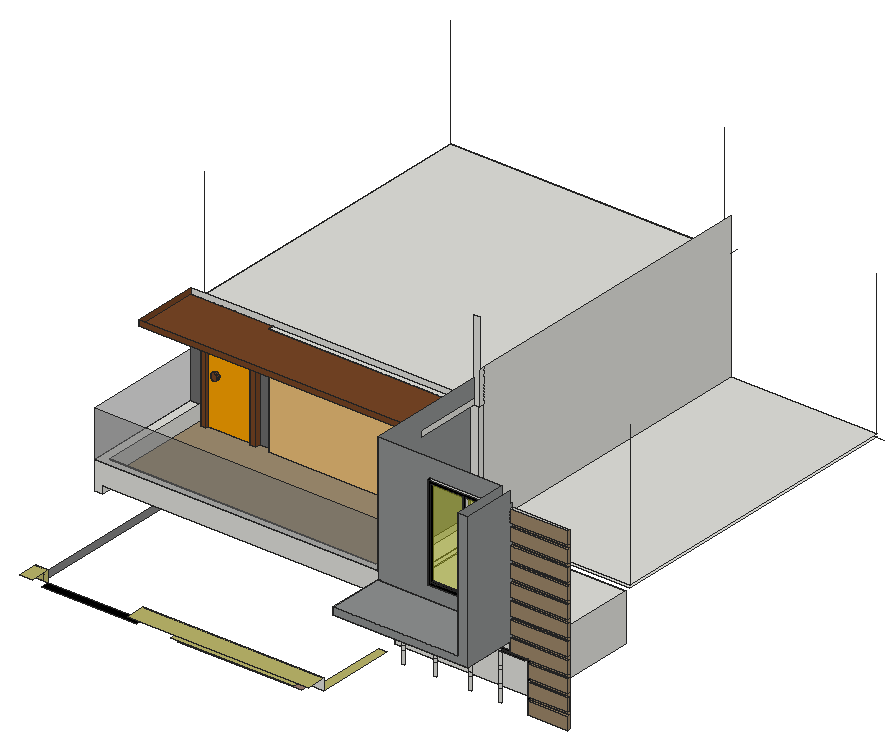
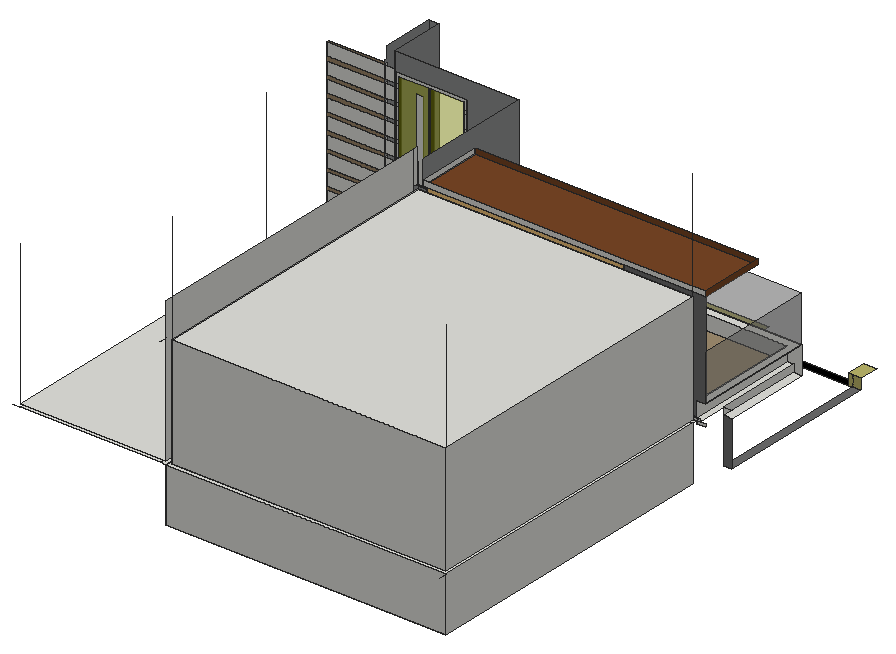
# SketchUp Ruby script. Lengths in inches.
U = 1.inch
M = Sketchup.active_model
def pt(a) = Geom::Point3d.new(a.map { |v| v * U })
def face(e, loops, mat)
  f = e.add_face(loops[0].map { |a| pt(a) })
  loops[1..].each { |l| e.add_face(l.map { |a| pt(a) }).erase! }
  f.material = f.back_material = mat if mat
  f
end
# faces: each face lists its corners as indices into pts; further lists are holes
def faces(e, pts, list, mat = nil) = list.each { |f| face(e, (f[0].is_a?(Array) ? f : [f]).map { |l| l.map { |i| pts[i] } }, mat) }
# xy, xz, yz: faces in a plane at the given z, y or x. An outline is a flat list of corners, or four numbers for a rectangle; further outlines are holes
def ring(l) = l.size == 4 ? [[l[0], l[1]], [l[2], l[1]], [l[2], l[3]], [l[0], l[3]]] : l.each_slice(2).to_a
def flat(e, list, mat, &to3) = list.each { |f| face(e, (f[0].is_a?(Array) ? f : [f]).map { |l| ring(l).map { |u, v| to3.(u, v) } }, mat) }
def xy(e, z, list, mat = nil) = flat(e, list, mat) { |x, y| [x, y, z] }
def xz(e, y, list, mat = nil) = flat(e, list, mat) { |x, z| [x, y, z] }
def yz(e, x, list, mat = nil) = flat(e, list, mat) { |y, z| [x, y, z] }
def lines(e, pts, list) = list.each { |a, b| e.add_line(pt(pts[a]), pt(pts[b])) }
# prism: a flat outline (further loops are holes) pulled along v
def prism(e, loops, v, mat = nil)
  f = face(e, loops, mat); d = Geom::Vector3d.new(v.map { |x| x * U })
  f.pushpull(f.normal.samedirection?(d) ? d.length : -d.length)
end
def box(e, o, s, mat = nil) = prism(e, [[o, [o[0] + s[0], o[1], o[2]], [o[0] + s[0], o[1] + s[1], o[2]], [o[0], o[1] + s[1], o[2]]]], [0, 0, s[2]], mat)
def at(x, y, z, deg = 0) = Geom::Transformation.translation(pt([x, y, z])) * Geom::Transformation.rotation(ORIGIN, Z_AXIS, deg.degrees)
def axes(o, x, y, z) = Geom::Transformation.new([*x, 0, *y, 0, *z, 0, *pt(o).to_a, 1])
def part(name) = M.definitions.add(name)
# library, detail: a bought-in or finely detailed component or shape, given as its bounding box
def library(name, o, s) = part(name).tap { |d| box(d.entities, o, s) }
def detail(e, o, s) = box(e.add_group.entities, o, s)
def put(e, d, t, mat = nil) = e.add_instance(d, t).tap { |i| i.material = mat if mat }
def group(e, t, mat = nil) = e.add_group.tap { |g| g.transformation = t; g.material = mat if mat }.entities
root = M.entities
M.materials.add("Niraj_Hair_Dark").color = [109, 109, 109]
M.materials.add("Niraj_Skin").color = [158, 128, 115]
M.materials.add("[0035_Tan]").color = [158, 135, 105]
M.materials.add("[0038_Orange]").color = [255, 165, 0]
M.materials.add("[0057_DarkKhaki]").color = [189, 183, 107]
M.materials.add("[0137_Black]").color = [0, 0, 0]
M.materials.add("[Blacktop Old 02]").color = [143, 145, 145]
M.materials.add("[Tile Border Travertine]").color = [160, 142, 112]
M.materials.add("[Translucent Glass Gray]").color = [198, 206, 26]
M.materials["[Translucent Glass Gray]"].alpha = 0.5
M.materials.add("[Translucent Glass Gray]1").color = [128, 128, 128]
M.materials["[Translucent Glass Gray]1"].alpha = 0.5
M.materials.add("[Wood OSB]").color = [240, 195, 122]
M.materials.add("[Wood Veneer 01]").color = [120, 70, 37]
box(root,[12.5,268.5,123],[297.6875,334,120])
xy(root,58.58,[[475.91,128.5,518.75,131.5]],"[0035_Tan]")
xy(root,60,[[3.5,51.8125,12.5,226.5]],"Niraj_Hair_Dark")
xy(root,60,[[166.59,40.8125,300.3,51.8125]],"Niraj_Skin")
xy(root,60,[[307.1875,51.8125,316.1875,137.32]],"[0057_DarkKhaki]")
xy(root,60,[[17,42.8125,119.91,51.8125]],"[0137_Black]")
xy(root,61.1875,[[12.5,268.5,316.1875,602.5]])
xy(root,67.8125,[[166.59,30.8125,300.3,51.8125]],"[0057_DarkKhaki]")
xy(root,68.75,[[322.1875,140.5,474.5,262.5]])
xy(root,72,[[3.5,30.8125,17,51.8125],[119.91,30.8125,316.1875,51.8125]],"[0057_DarkKhaki]")
xy(root,72.4375,[[475.91,128.5,518.75,131.5]],"[0035_Tan]")
xy(root,76.58,[[475.91,131.25,518.75,131.5]])
xy(root,76.58,[[475.91,128.5,518.75,131.25]],"[0035_Tan]")
xy(root,84,[[194.48,259.5,242.48,262.5]])
xy(root,84,[[194.48,256.5,242.48,259.5]],"[Wood Veneer 01]")
xy(root,90,[[188.48,256.5,248.48,262.5]],"[Wood Veneer 01]")
xy(root,90.4375,[[475.91,131.25,518.75,131.5]])
xy(root,90.4375,[[475.91,128.5,518.75,131.25]],"[0035_Tan]")
xy(root,94.58,[[475.91,128.5,518.75,131.5]],"[0035_Tan]")
xy(root,108.4375,[[475.91,128.5,518.75,131.5]],"[0035_Tan]")
xy(root,109.4375,[[3.5,131.5,12.5,226.5]])
xy(root,110.09,[[340.16,128.5,371.84,131.5],[374.84,128.5,409.66,131.5],[412.66,128.5,442.41,131.5],[445.41,128.5,472.91,131.5]],"[0137_Black]")
xy(root,112.58,[[475.91,128.5,518.75,131.5]],"[0035_Tan]")
xy(root,113.09,[[456.23,128.5,475.91,131.5]])
xy(root,113.09,[[337.16,128.5,456.23,131.5]],"[0137_Black]")
xy(root,117.125,[[12.5,131.5,12.5,256.5,20.37,256.5,20.37,259.5,23.875,259.5,23.875,256.5,31.74,256.5,31.74,259.5,35.25,259.5,35.25,256.5,43.12,256.5,43.12,259.5,46.625,259.5,46.625,256.5,54.49,256.5,54.49,259.5,58,259.5,58,256.5,65.87,256.5,65.87,259.5,69.375,259.5,69.375,256.5,77.24,256.5,77.24,259.5,80.75,259.5,80.75,256.5,88.62,256.5,88.62,259.5,92.125,259.5,92.125,256.5,99.99,256.5,99.99,259.5,103.5,259.5,103.5,256.5,111.37,256.5,111.37,259.5,114.875,259.5,114.875,256.5,122.74,256.5,122.74,259.5,126.25,259.5,126.25,256.5,134.12,256.5,134.12,259.5,137.625,259.5,137.625,256.5,147.33,256.5,147.33,262.5,316.1875,262.5,316.1875,131.5],[12.5,256.5,20.37,259.5],[23.875,256.5,31.74,259.5],[35.25,256.5,43.12,259.5],[46.625,256.5,54.49,259.5],
  [58,256.5,65.87,259.5],[69.375,256.5,77.24,259.5],[80.75,256.5,88.62,259.5],[92.125,256.5,99.99,259.5],[103.5,256.5,111.37,259.5],
  [114.875,256.5,122.74,259.5],[126.25,256.5,134.12,259.5],[137.625,256.5,145.49,259.5],[145.49,256.5,147.33,259.5]])
xy(root,120,[[316.1875,140.5,322.1875,262.5],[322.1875,140.5,474.5,262.5],[12.5,259.5,147.33,262.5],[12.5,262.5,316.1875,268.5],[12.5,268.5,316.1875,602.5],
  [316.1875,268.5,322.1875,602.5],[322.1875,268.5,474.5,602.5]])
xy(root,123,[[18.33,256.5,24.33,262.5],[72.33,256.5,78.33,262.5],[24.33,259.5,72.33,262.5],[316.1875,268.5,474.5,602.5]])
xy(root,123,[[310.1875,71.5,456.23,131.5]],"[Blacktop Old 02]")
xy(root,123,[[12.5,140.5,301.1875,140.5,301.1875,256.5,92.19,256.5,92.19,262.5,78.33,262.5,78.33,256.5,72.33,256.5,72.33,259.5,24.33,259.5,24.33,256.5,18.33,256.5,18.33,262.5,12.5,262.5]],"[Tile Border Travertine]")
xy(root,126.4375,[[456.23,128.5,518.75,131.5]],"[0035_Tan]")
xy(root,130.58,[[456.23,128.5,518.75,131.5]],"[0035_Tan]")
xy(root,130.65,[[310.1875,71.5,445.29,131.5]],"[Blacktop Old 02]")
xy(root,139.125,[[3.5,131.5,310.1875,131.5,310.1875,256.5,301.1875,256.5,301.1875,140.5,12.5,140.5,12.5,262.5,3.5,262.5],[301.1875,256.5,310.1875,262.5]])
xy(root,144.4375,[[456.23,128.5,518.75,131.5]],"[0035_Tan]")
xy(root,147.46,[[367.23,128.5,444.17,131.5]],"[0137_Black]")
xy(root,148.58,[[456.23,128.5,518.75,131.5]])
xy(root,150.46,[[370.23,128.5,405.7,131.5],[408.7,128.5,441.17,131.5]],"[0137_Black]")
xy(root,162.4375,[[456.23,128.5,518.75,131.5]],"[0035_Tan]")
xy(root,166.58,[[456.23,128.5,518.75,131.5]])
xy(root,180.4375,[[456.23,128.5,518.75,131.5]],"[0035_Tan]")
xy(root,184.58,[[456.23,128.5,518.75,131.5]])
xy(root,198.4375,[[456.23,128.5,518.75,131.5]],"[0035_Tan]")
xy(root,202.58,[[456.23,128.5,518.75,131.5]])
xy(root,207,[[24.33,256.5,72.33,259.5]],"[Wood Veneer 01]")
xy(root,213,[[18.33,256.5,78.33,262.5]],"[Wood Veneer 01]")
xy(root,216.4375,[[456.23,128.5,518.75,131.5]],"[0035_Tan]")
xy(root,220.58,[[456.23,128.5,518.75,131.5]],"[0035_Tan]")
xy(root,234.4375,[[456.23,128.5,518.75,131.5]],"[0035_Tan]")
xy(root,238.58,[[456.23,128.5,518.75,131.5]],"[0035_Tan]")
xy(root,243,[[92.19,256.5,310.1875,262.5]])
xy(root,243,[[3.5,191.32,3.5,262.5,92.19,262.5,92.19,256.5,310.1875,256.5,310.1875,191.32]],"[Wood Veneer 01]")
xy(root,246.27,[[370.23,128.5,405.7,131.5],[408.7,128.5,441.17,131.5]],"[0137_Black]")
xz(root,51.8125,[[300.3,60,300.3,67.8125,166.59,67.8125,166.59,72,316.1875,72,316.1875,60]])
xz(root,51.8125,[[3.5,60,12.5,72],[12.5,60,17,72],[119.91,60,166.59,72]],"[0057_DarkKhaki]")
xz(root,71.5,[[310.1875,123,456.23,123,456.23,269.38,445.29,269.38,445.29,130.65,310.1875,130.65]],"[Blacktop Old 02]")
xz(root,128.5,[[475.91,58.58,518.75,72.4375],[475.91,76.58,518.75,90.4375],[475.91,94.58,518.75,108.4375],[475.91,112.58,518.75,112.58,518.75,126.4375,456.23,126.4375,456.23,113.09,475.91,113.09],[456.23,130.58,518.75,144.4375],
  [456.23,148.58,518.75,162.4375],[456.23,166.58,518.75,180.4375],[456.23,184.58,518.75,198.4375],[456.23,202.58,518.75,216.4375],[456.23,220.58,518.75,234.4375],
  [456.23,238.58,518.75,252.4375]],"[0035_Tan]")
xz(root,128.5,[[[367.23,147.46,444.17,249.27],[370.23,150.46,405.7,246.27],[408.7,150.46,441.17,246.27]]],"[0137_Black]")
xz(root,131.25,[[475.91,76.58,518.75,90.4375]])
xz(root,131.5,[[337.16,58.58,340.16,72.4375],[371.84,58.58,374.84,72.4375],[409.66,58.58,412.66,72.4375],[442.41,58.58,445.41,72.4375],[472.91,58.58,475.91,72.4375],
  [475.91,58.58,518.75,72.4375],[337.16,72.4375,340.16,76.58],[371.84,72.4375,374.84,76.58],[409.66,72.4375,412.66,76.58],[442.41,72.4375,445.41,76.58],
  [472.91,72.4375,475.91,76.58],[337.16,76.58,340.16,90.4375],[371.84,76.58,374.84,90.4375],[409.66,76.58,412.66,90.4375],[442.41,76.58,445.41,90.4375],
  [472.91,76.58,475.91,90.4375],[475.91,76.58,518.75,90.4375],[337.16,90.4375,340.16,94.58],[371.84,90.4375,374.84,94.58],[409.66,90.4375,412.66,94.58],
  [442.41,90.4375,445.41,94.58],[472.91,90.4375,475.91,94.58],[337.16,94.58,340.16,108.4375],[371.84,94.58,374.84,108.4375],[409.66,94.58,412.66,108.4375],
  [442.41,94.58,445.41,108.4375],[472.91,94.58,475.91,108.4375],[475.91,94.58,518.75,108.4375],[337.16,108.4375,337.16,112.58,475.91,112.58,475.91,108.4375,472.91,108.4375,472.91,110.09,445.41,110.09,445.41,108.4375,442.41,108.4375,442.41,110.09,412.66,110.09,412.66,108.4375,409.66,108.4375,409.66,110.09,374.84,110.09,374.84,108.4375,371.84,108.4375,371.84,110.09,340.16,110.09,340.16,108.4375],[3.5,109.4375,12.5,109.4375,12.5,117.125,316.1875,117.125,316.1875,123,310.1875,123,310.1875,139.125,3.5,139.125],
  [337.16,112.58,475.91,113.09],[475.91,112.58,475.91,113.09,456.23,113.09,456.23,126.4375,518.75,126.4375,518.75,112.58],[310.1875,123,456.23,126.4375],[310.1875,130.58,456.23,130.58,456.23,144.4375,445.29,144.4375,445.29,130.65,310.1875,130.65],[456.23,130.58,518.75,144.4375],
  [367.23,147.46,444.17,148.58],[367.23,148.58,444.17,148.58,444.17,162.4375,441.17,162.4375,441.17,150.46,408.7,150.46,408.7,162.4375,405.7,162.4375,405.7,150.46,370.23,150.46,370.23,162.4375,367.23,162.4375],[444.17,148.58,445.29,162.4375],[445.29,148.58,456.23,162.4375],[456.23,148.58,518.75,162.4375],
  [367.23,162.4375,370.23,166.58],[405.7,162.4375,408.7,166.58],[441.17,162.4375,444.17,166.58],[444.17,162.4375,445.29,166.58],[367.23,166.58,370.23,180.4375],
  [405.7,166.58,408.7,180.4375],[441.17,166.58,444.17,180.4375],[444.17,166.58,445.29,180.4375],[445.29,166.58,456.23,180.4375],[456.23,166.58,518.75,180.4375],
  [367.23,180.4375,370.23,184.58],[405.7,180.4375,408.7,184.58],[441.17,180.4375,444.17,184.58],[444.17,180.4375,445.29,184.58],[367.23,184.58,370.23,198.4375],
  [405.7,184.58,408.7,198.4375],[441.17,184.58,444.17,198.4375],[444.17,184.58,445.29,198.4375],[445.29,184.58,456.23,198.4375],[456.23,184.58,518.75,198.4375],
  [367.23,198.4375,370.23,202.58],[405.7,198.4375,408.7,202.58],[441.17,198.4375,444.17,202.58],[444.17,198.4375,445.29,202.58],[367.23,202.58,370.23,216.4375],
  [405.7,202.58,408.7,216.4375],[441.17,202.58,444.17,216.4375],[444.17,202.58,445.29,216.4375],[445.29,202.58,456.23,216.4375],[456.23,202.58,518.75,216.4375],
  [367.23,216.4375,370.23,220.58],[405.7,216.4375,408.7,220.58],[441.17,216.4375,444.17,220.58],[444.17,216.4375,445.29,220.58],[367.23,220.58,370.23,234.4375],
  [405.7,220.58,408.7,234.4375],[441.17,220.58,444.17,234.4375],[444.17,220.58,445.29,234.4375],[445.29,220.58,456.23,234.4375],[456.23,220.58,518.75,234.4375],
  [367.23,234.4375,370.23,238.58],[405.7,234.4375,408.7,238.58],[441.17,234.4375,444.17,238.58],[444.17,234.4375,445.29,238.58],[367.23,238.58,370.23,238.58,370.23,246.27,405.7,246.27,405.7,238.58,408.7,238.58,408.7,246.27,441.17,246.27,441.17,238.58,444.17,238.58,444.17,249.27,367.23,249.27],
  [445.29,238.58,456.23,252.4375],[456.23,238.58,518.75,252.4375]])
xz(root,131.5,[[475.91,72.4375,518.75,76.58],[475.91,90.4375,518.75,94.58],[475.91,108.4375,518.75,112.58],[456.23,126.4375,518.75,130.58],[456.23,144.4375,518.75,148.58],
  [456.23,162.4375,518.75,166.58],[456.23,180.4375,518.75,184.58],[456.23,198.4375,518.75,202.58],[456.23,216.4375,518.75,220.58],[456.23,234.4375,518.75,238.58]],"[0035_Tan]")
xz(root,131.5,[[310.1875,130.65,445.29,130.65,445.29,148.58,444.17,148.58,444.17,147.46,367.23,147.46,367.23,249.27,444.17,249.27,444.17,238.58,445.29,238.58,445.29,269.38,310.1875,269.38]],"[Blacktop Old 02]")
xz(root,131.5,[[370.23,150.46,405.7,246.27],[408.7,150.46,441.17,246.27]],"[Translucent Glass Gray]")
xz(root,131.5,[[3.5,139.125,310.1875,189.71]],"[Translucent Glass Gray]1")
xz(root,140.5,[[322.1875,68.75,474.5,120],[12.5,123,301.1875,139.125]])
xz(root,191.32,[[3.5,243,310.1875,249.09]],"[Wood Veneer 01]")
xz(root,226.5,[[3.5,60,12.5,109.4375]],"Niraj_Hair_Dark")
xz(root,256.5,[[92.19,123,301.1875,123,301.1875,139.125,310.1875,139.125,310.1875,243,92.19,243]],"[Wood OSB]")
xz(root,256.5,[[18.33,123,24.33,123,24.33,207,72.33,207,72.33,123,78.33,123,78.33,213,18.33,213],[32.84,171.39,33.83,171.52,34.75,171.9,35.54,172.51,36.14,173.3,36.52,174.22,36.65,175.2,36.52,176.19,36.14,177.11,35.54,177.9,34.75,178.51,33.83,178.89,32.84,179.02,31.85,178.89,30.93,178.51,30.15,177.9,29.54,177.11,29.16,176.19,29.03,175.2,29.16,174.22,29.54,173.3,30.15,172.51,30.93,171.9,31.85,171.52]],"[Wood Veneer 01]")
xz(root,259.5,[[12.5,117.125,147.33,120]])
xz(root,259.5,[[[24.33,123,72.33,207],[32.84,171.39,31.85,171.52,30.93,171.9,30.15,172.51,29.54,173.3,29.16,174.22,29.03,175.2,29.16,176.19,29.54,177.11,30.15,177.9,30.93,178.51,31.85,178.89,32.84,179.02,33.83,178.89,34.75,178.51,35.54,177.9,36.14,177.11,36.52,176.19,36.65,175.2,36.52,174.22,36.14,173.3,35.54,172.51,34.75,171.9,33.83,171.52]]],"[0038_Orange]")
xz(root,262.5,[[322.1875,68.75,474.5,120],[18.33,117,78.33,120],[3.5,117.125,12.5,120],[147.33,117.125,316.1875,120],[12.5,120,18.33,123],
  [18.33,120,78.33,123],[301.1875,123,310.1875,139.125],[3.5,243,3.5,249.09,18.5,249.09,18.5,249,71.22,249,71.22,249.09,310.1875,249.09,310.1875,243],[310.1875,243,316.1875,330.3125]])
xz(root,262.5,[[12.5,123,18.33,123,18.33,213,78.33,213,78.33,123,92.19,123,92.19,243,3.5,243,3.5,139.125,12.5,139.125]],"Niraj_Hair_Dark")
xz(root,268.5,[[12.5,61.1875,316.1875,120]])
xz(root,602.5,[[12.5,61.1875,316.1875,120]])
yz(root,3.5,[[131.5,139.125,262.5,189.71]],"[Translucent Glass Gray]1")
yz(root,3.5,[[191.32,243,262.5,249.09]],"[Wood Veneer 01]")
yz(root,12.5,[[268.5,61.1875,602.5,120],[131.5,109.4375,226.5,117.125],[259.5,117.125,262.5,120],[140.5,123,262.5,139.125]])
yz(root,18.33,[[256.5,123,262.5,213]],"[Wood Veneer 01]")
yz(root,24.33,[[256.5,123,259.5,207]],"[Wood Veneer 01]")
yz(root,72.33,[[256.5,123,259.5,207]],"[Wood Veneer 01]")
yz(root,78.33,[[256.5,123,262.5,213]],"[Wood Veneer 01]")
yz(root,92.19,[[256.5,123,262.5,243]],"Niraj_Hair_Dark")
yz(root,147.33,[[259.5,117.125,262.5,120]])
yz(root,301.1875,[[140.5,123,256.5,139.125],[256.5,123,262.5,139.125]])
yz(root,310.1875,[[71.5,123,131.5,130.65],[191.32,243,262.5,249.09]])
yz(root,310.1875,[[131.5,139.125,131.5,269.38,262.5,269.38,262.5,249.09,191.32,249.09,191.32,243,256.5,243,256.5,139.125]],"[Blacktop Old 02]")
yz(root,316.1875,[[268.5,61.1875,602.5,120],[140.5,117.125,262.5,120],[268.5,123,602.5,279],[262.5,243,268.5,279]])
yz(root,322.1875,[[140.5,68.75,262.5,120]])
yz(root,367.23,[[128.5,147.46,131.5,249.27]],"[0137_Black]")
yz(root,370.23,[[128.5,150.46,131.5,246.27]],"[0137_Black]")
yz(root,405.7,[[128.5,150.46,131.5,246.27]],"[0137_Black]")
yz(root,408.7,[[128.5,150.46,131.5,246.27]])
yz(root,441.17,[[128.5,150.46,131.5,246.27]],"[0137_Black]")
yz(root,444.17,[[128.5,147.46,131.5,249.27]])
yz(root,445.29,[[71.5,130.65,131.5,269.38]],"[Blacktop Old 02]")
yz(root,456.23,[[128.5,113.09,131.5,123],[128.5,123,131.5,126.4375],[128.5,130.58,131.5,144.4375],[128.5,148.58,131.5,162.4375],[128.5,166.58,131.5,180.4375],
  [128.5,184.58,131.5,198.4375],[128.5,202.58,131.5,216.4375],[128.5,220.58,131.5,234.4375],[128.5,238.58,131.5,252.4375]])
yz(root,456.23,[[71.5,123,128.5,123,128.5,126.4375,131.5,126.4375,131.5,130.58,128.5,130.58,128.5,144.4375,131.5,144.4375,131.5,148.58,128.5,148.58,128.5,162.4375,131.5,162.4375,131.5,166.58,128.5,166.58,128.5,180.4375,131.5,180.4375,131.5,184.58,128.5,184.58,128.5,198.4375,131.5,198.4375,131.5,202.58,128.5,202.58,128.5,216.4375,131.5,216.4375,131.5,220.58,128.5,220.58,128.5,234.4375,131.5,234.4375,131.5,238.58,128.5,238.58,128.5,252.4375,131.5,252.4375,131.5,256.58,128.5,256.58,128.5,269.38,71.5,269.38]],"[Blacktop Old 02]")
yz(root,474.5,[[140.5,68.75,262.5,120]])
yz(root,475.91,[[128.5,58.58,131.5,72.4375],[128.5,76.58,131.25,90.4375],[131.25,76.58,131.5,90.4375],[128.5,94.58,131.5,108.4375],[128.5,112.58,131.5,113.09]])
yz(root,475.91,[[128.5,72.4375,131.5,76.58],[128.5,90.4375,131.5,94.58],[128.5,108.4375,131.5,112.58]],"[0137_Black]")
yz(root,518.75,[[131.25,76.58,131.5,90.4375]])
yz(root,518.75,[[128.5,58.58,131.5,72.4375],[128.5,76.58,131.25,90.4375],[128.5,94.58,131.5,108.4375],[128.5,112.58,131.5,126.4375],[128.5,130.58,131.5,144.4375],
  [128.5,148.58,131.5,162.4375],[128.5,166.58,131.5,180.4375],[128.5,184.58,131.5,198.4375],[128.5,202.58,131.5,216.4375],[128.5,220.58,131.5,234.4375],
  [128.5,238.58,131.5,252.4375]],"[0035_Tan]")
p = [[31.85,259.5,171.52],[32.84,259.5,171.39],[32.84,256.5,171.39],[31.85,256.5,171.52],[33.83,259.5,171.52],[33.83,256.5,171.52],
  [30.93,259.5,171.9],[30.93,256.5,171.9],[34.75,259.5,171.9],[34.75,256.5,171.9],[30.15,259.5,172.51],[30.15,256.5,172.51],
  [35.54,259.5,172.51],[35.54,256.5,172.51],[29.54,259.5,173.3],[29.54,256.5,173.3],[36.14,259.5,173.3],[36.14,256.5,173.3],
  [29.16,259.5,174.22],[29.16,256.5,174.22],[36.52,259.5,174.22],[36.52,256.5,174.22],[29.03,259.5,175.2],[29.03,256.5,175.2],
  [36.65,259.5,175.2],[36.65,256.5,175.2],[29.16,259.5,176.19],[29.16,256.5,176.19],[36.52,259.5,176.19],[36.52,256.5,176.19],
  [29.54,259.5,177.11],[29.54,256.5,177.11],[36.14,259.5,177.11],[36.14,256.5,177.11],[30.15,259.5,177.9],[30.15,256.5,177.9],
  [35.54,259.5,177.9],[35.54,256.5,177.9],[30.93,259.5,178.51],[30.93,256.5,178.51],[34.75,259.5,178.51],[34.75,256.5,178.51],
  [31.85,259.5,178.89],[31.85,256.5,178.89],[33.83,259.5,178.89],[33.83,256.5,178.89],[32.84,259.5,179.02],[32.84,256.5,179.02],
  [12.5,602.5,120],[12.5,611.5,120],[474.5,602.5,120],[483.5,602.5,120],[474.5,268.5,123],[474.5,268.5,279],
  [474.5,602.5,123],[474.5,602.5,279],[316.1875,611.5,243],[316.1875,602.5,243],[310.1875,602.5,243],[310.1875,602.5,363],
  [12.5,602.5,243],[12.5,602.5,363],[310.1875,268.5,243],[310.1875,268.5,269.38],[12.5,268.5,243],[12.5,268.5,363],
  [3.5,226.5,117.125],[12.5,226.5,117.125],[300.3,42,67.8125],[307.1875,42,67.8125]]
faces(root,p,[[0,1,2,3],[1,4,5,2],[6,0,3,7],[4,8,9,5],[10,6,7,11],[8,12,13,9],[14,10,11,15],[12,16,17,13],
  [18,14,15,19],[16,20,21,17],[22,18,19,23],[20,24,25,21],[26,22,23,27],[24,28,29,25],[30,26,27,31],[28,32,33,29],
  [34,30,31,35],[32,36,37,33],[38,34,35,39],[36,40,41,37],[42,38,39,43],[40,44,45,41],[46,42,43,47],[44,46,47,45]],"[Wood Veneer 01]")
lines(root,p,[[48,49],[50,51],[52,53],[54,55],[56,57],[58,59],[60,61],[62,63],[64,65],[66,67],[68,69]])
